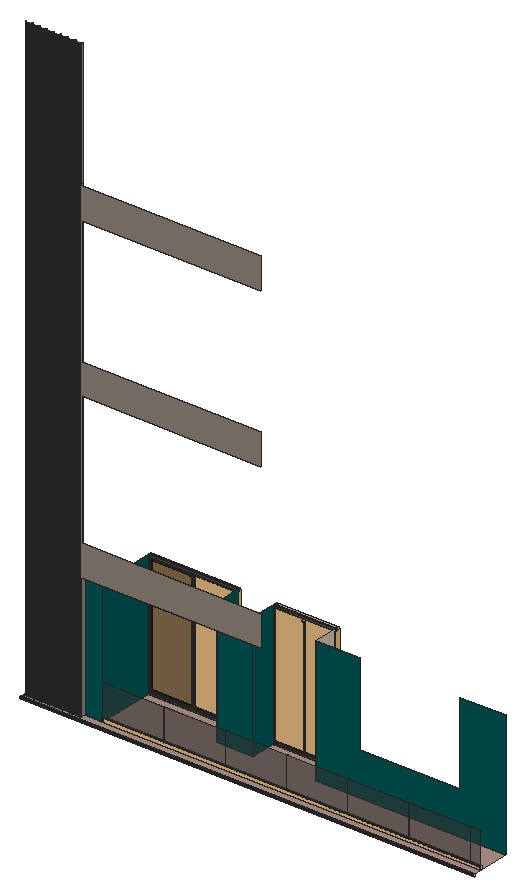
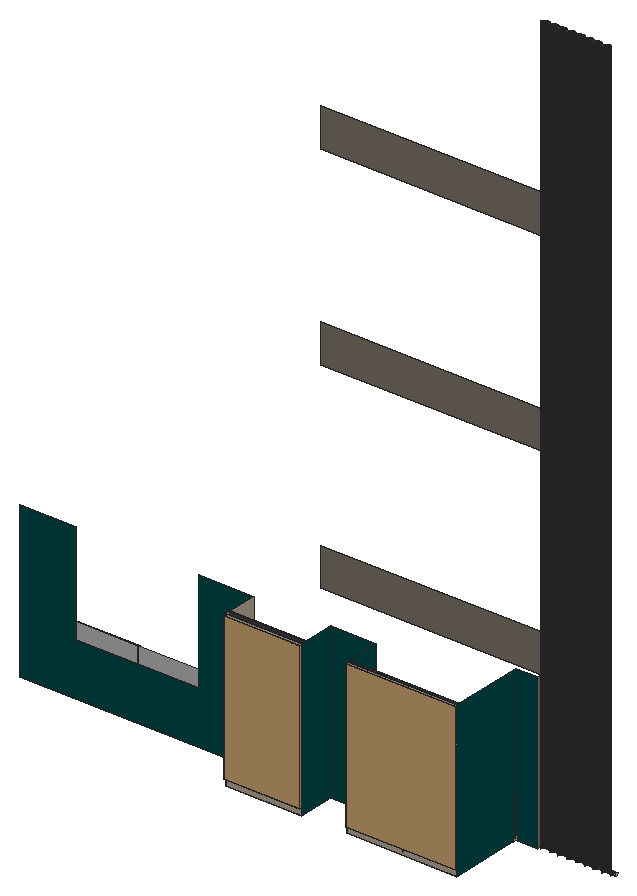
# SketchUp Ruby script. Lengths in inches.
U = 1.inch
M = Sketchup.active_model
def pt(a) = Geom::Point3d.new(a.map { |v| v * U })
def face(e, loops, mat)
  f = e.add_face(loops[0].map { |a| pt(a) })
  loops[1..].each { |l| e.add_face(l.map { |a| pt(a) }).erase! }
  f.material = f.back_material = mat if mat
  f
end
# faces: each face lists its corners as indices into pts; further lists are holes
def faces(e, pts, list, mat = nil) = list.each { |f| face(e, (f[0].is_a?(Array) ? f : [f]).map { |l| l.map { |i| pts[i] } }, mat) }
# xy, xz, yz: faces in a plane at the given z, y or x. An outline is a flat list of corners, or four numbers for a rectangle; further outlines are holes
def ring(l) = l.size == 4 ? [[l[0], l[1]], [l[2], l[1]], [l[2], l[3]], [l[0], l[3]]] : l.each_slice(2).to_a
def flat(e, list, mat, &to3) = list.each { |f| face(e, (f[0].is_a?(Array) ? f : [f]).map { |l| ring(l).map { |u, v| to3.(u, v) } }, mat) }
def xy(e, z, list, mat = nil) = flat(e, list, mat) { |x, y| [x, y, z] }
def xz(e, y, list, mat = nil) = flat(e, list, mat) { |x, z| [x, y, z] }
def yz(e, x, list, mat = nil) = flat(e, list, mat) { |y, z| [x, y, z] }
def lines(e, pts, list) = list.each { |a, b| e.add_line(pt(pts[a]), pt(pts[b])) }
# prism: a flat outline (further loops are holes) pulled along v
def prism(e, loops, v, mat = nil)
  f = face(e, loops, mat); d = Geom::Vector3d.new(v.map { |x| x * U })
  f.pushpull(f.normal.samedirection?(d) ? d.length : -d.length)
end
def box(e, o, s, mat = nil) = prism(e, [[o, [o[0] + s[0], o[1], o[2]], [o[0] + s[0], o[1] + s[1], o[2]], [o[0], o[1] + s[1], o[2]]]], [0, 0, s[2]], mat)
def at(x, y, z, deg = 0) = Geom::Transformation.translation(pt([x, y, z])) * Geom::Transformation.rotation(ORIGIN, Z_AXIS, deg.degrees)
def axes(o, x, y, z) = Geom::Transformation.new([*x, 0, *y, 0, *z, 0, *pt(o).to_a, 1])
def part(name) = M.definitions.add(name)
# library, detail: a bought-in or finely detailed component or shape, given as its bounding box
def library(name, o, s) = part(name).tap { |d| box(d.entities, o, s) }
def detail(e, o, s) = box(e.add_group.entities, o, s)
def put(e, d, t, mat = nil) = e.add_instance(d, t).tap { |i| i.material = mat if mat }
def group(e, t, mat = nil) = e.add_group.tap { |g| g.transformation = t; g.material = mat if mat }.entities
root = M.entities
M.materials.add("Brown Tiles 240cm").color = [174, 145, 135]
M.materials.add("Glass_Tinted_Gray").color = [0, 0, 0]
M.materials["Glass_Tinted_Gray"].alpha = 0.125
M.materials.add("Heather_Band").color = [142, 133, 122]
M.materials.add("Lily_Blonde").color = [209, 194, 173]
M.materials.add("[0135_DarkGray]").color = [81, 81, 81]
M.materials.add("[Color H08]").color = [0, 84, 84]
M.materials.add("[Mirror 02]").color = [229, 229, 229]
M.materials.add("[Terrazzo Light Blue]").color = [196, 214, 227]
M.materials.add("[Translucent_Glass_Blue]").color = [63, 63, 63]
M.materials["[Translucent_Glass_Blue]"].alpha = 0.35
M.materials.add("metal railing").color = [165, 165, 165]
M.materials.add("plastic2").color = [86, 86, 86]
c1 = library("Window curtains",[0,0,0],[14.46,147.43,135.83])
c2 = part("PENTEK_RP Fineline 50S_Sliding_DoorCase_E1")
box(c2.entities,[0,0,0],[1.51,3.66,99.27],"[0135_DarkGray]")
c3 = part("PENTEK_RP Fineline 50S_SlidingDooe_Case_E2")
box(c3.entities,[0,0,0],[96.25,3.66,1.51],"[0135_DarkGray]")
c4 = part("pentek_RP Fineline 50S_SlidingDoor_Case")
put(c4.entities,c2,at(97.76,0,0))
put(c4.entities,c3,at(1.51,0,0))
put(c4.entities,c2,at(0,0,0))
put(c4.entities,c3,at(1.51,0,97.76))
c5 = part("PENTEK_RP Fineline 50S_SlidingDoor_GlazingBead_2")
box(c5.entities,[0,0,0],[0.56,0.59,94.39],"[0135_DarkGray]")
c6 = part("PENTEK_RP Fineline 50S_SlidingDoor_Glass")
box(c6.entities,[0,0,0],[46.58,0.16,94.39],"Glass_Tinted_Gray")
c7 = part("PENTEK_RP Fineline 50S_SlidingDoor_GlazingBead")
box(c7.entities,[0,0,0],[45.47,0.59,0.56],"[0135_DarkGray]")
c8 = part("PENTEK_RP Fineline 50S_SlidingDoor_Leaf_E1")
xy(c8.entities,0,[[0,0,0.93,1.97],[0.93,1.57,1.49,1.97]],"[0135_DarkGray]")
xy(c8.entities,96.25,[[0,0,0.93,0,0.93,1.57,1.49,1.57,1.49,1.97,0,1.97]],"[0135_DarkGray]")
xz(c8.entities,0,[[0,0,0.93,96.25]],"[0135_DarkGray]")
xz(c8.entities,1.57,[[0.93,0,1.49,95.32],[0.93,95.32,1.49,96.25]],"[0135_DarkGray]")
xz(c8.entities,1.97,[[0,0,1.49,96.25]],"[0135_DarkGray]")
yz(c8.entities,0,[[0,0,1.97,96.25]],"[0135_DarkGray]")
yz(c8.entities,0.93,[[0,0,1.57,0.93],[0,0.93,1.57,95.32],[0,95.32,1.57,96.25]],"[0135_DarkGray]")
yz(c8.entities,1.49,[[1.57,0,1.97,95.32],[1.57,95.32,1.97,96.25]],"[0135_DarkGray]")
c9 = part("PENTEK_RP Fineline 50S_SlidingDoor_Leaf_E2")
xy(c9.entities,0,[[0,0,0,1.57,0.56,1.57,0.56,1.97,46.02,1.97,46.02,1.57,46.58,1.57,46.58,0]],"[0135_DarkGray]")
xy(c9.entities,0.93,[[0,0,46.58,1.57]],"[0135_DarkGray]")
xy(c9.entities,1.49,[[0.56,1.57,46.02,1.97]],"[0135_DarkGray]")
xz(c9.entities,0,[[0,0,46.58,0.93]],"[0135_DarkGray]")
xz(c9.entities,1.57,[[0,0,0.56,0.93],[46.02,0,46.58,0.93],[0.56,0.93,46.02,1.49]],"[0135_DarkGray]")
xz(c9.entities,1.97,[[0.56,0,46.02,1.49]],"[0135_DarkGray]")
yz(c9.entities,0,[[0,0,1.57,0.93]],"[0135_DarkGray]")
yz(c9.entities,0.56,[[1.57,0,1.97,0.93],[1.57,0.93,1.97,1.49]],"[0135_DarkGray]")
yz(c9.entities,46.02,[[1.57,0,1.97,0.93],[1.57,0.93,1.97,1.49]],"[0135_DarkGray]")
yz(c9.entities,46.58,[[0,0,1.57,0.93]],"[0135_DarkGray]")
c10 = part("PENTEK_RP Fineline S_SlidingDoor_Leaf1")
put(c10.entities,c5,at(0.93,0,0.93))
put(c10.entities,c5,at(46.96,0,0.93))
put(c10.entities,c6,at(1.49,1.42,0.93))
put(c10.entities,c7,at(1.49,0,0.93))
put(c10.entities,c6,at(1.49,0.59,0.93),"[Terrazzo Light Blue]")
put(c10.entities,c8,at(0,0,0))
put(c10.entities,c8,axes([48.44,0,0],[-1,0,0],[0,1,0],[0,0,1]))
put(c10.entities,c9,axes([0.93,0,96.25],[1,0,0],[0,1,0],[0,0,-1]))
put(c10.entities,c9,at(0.93,0,0))
put(c10.entities,c7,at(1.49,0,94.77))
c11 = part("PENTEK_RP Fineline 50S_SlidingDoor_Leaf2")
put(c11.entities,c6,at(1.49,1.42,0.93))
put(c11.entities,c7,at(1.49,0,94.77))
put(c11.entities,c5,at(46.96,0,0.93))
put(c11.entities,c6,at(1.49,0.59,0.93),"[Mirror 02]")
put(c11.entities,c5,at(0.93,0,0.93))
put(c11.entities,c8,at(0,0,0))
put(c11.entities,c8,axes([48.44,0,0],[-1,0,0],[0,1,0],[0,0,1]))
put(c11.entities,c7,at(1.49,0,0.93))
put(c11.entities,c9,axes([0.93,0,96.25],[1,0,0],[0,1,0],[0,0,-1]))
put(c11.entities,c9,at(0.93,0,0))
c12 = part("PENTEK - Slimmest Steel Sliding Door / Window\#1")
put(c12.entities,c4,at(0,-1.88,-0.09))
put(c12.entities,c10,at(1.51,-2.27,1.42))
put(c12.entities,c11,at(49.32,-0.3,1.42))
c13 = library("Railing",[0,0,0],[72,2.52,4.03])
c14 = part("railing plastic")
box(c14.entities,[0,0.75,0],[72,0.26,0.68],"plastic2")
box(c14.entities,[0,0,0],[72,0.26,0.68],"plastic2")
c15 = part("Glass Railing pro")
put(c15.entities,c13,axes([0,0,0],[6.18776,0,0],[0,1,0],[0,0,1]))
put(c15.entities,c14,axes([0,0.75,3.47],[6.18776,0,0],[0,1,0],[0,0,1]))
c16 = part("sheet glass")
box(c16.entities,[0,0,0],[39.37,0.39,39.37],"[Translucent_Glass_Blue]")
c17 = part("glass stretch")
box(c17.entities,[0,0,0],[39.37,0.39,43.31],"[Translucent_Glass_Blue]")
c18 = part("glass frame")
put(c18.entities,c16,axes([0,0,0],[1.8288,0,0],[0,1.016,0],[0,0,1]))
put(c18.entities,c17,axes([433.2,0,0],[0.3129,0,0],[0,1.016,0],[0,0,0.90909]))
put(c18.entities,c16,axes([72.2,0,0],[1.8288,0,0],[0,1.016,0],[0,0,1]))
put(c18.entities,c16,axes([144.4,0,0],[1.8288,0,0],[0,1.016,0],[0,0,1]))
put(c18.entities,c16,axes([216.6,0,0],[1.8288,0,0],[0,1.016,0],[0,0,1]))
put(c18.entities,c16,axes([288.8,0,0],[1.8288,0,0],[0,1.016,0],[0,0,1]))
put(c18.entities,c16,axes([361,0,0],[1.8288,0,0],[0,1.016,0],[0,0,1]))
c19 = part("Glass Railing +")
put(c19.entities,c15,at(0,0,0),"metal railing")
put(c19.entities,c18,at(0,1.0625,1.53),"metal railing")
c20 = part("My+Glass_Railing")
put(c20.entities,c19,at(-0.29,0,0))
c21 = part("Group\#18")
put(c21.entities,c1,axes([0,8.14,5.43],[0,-0.42,0],[1.40442,0,0],[0,0,0.9702]))
put(c21.entities,c12,axes([0,2.27,0.13],[2.0736,0,0],[0,1,0],[0,0,1.4]))
xy(root,219.25,[[0,1.33,534.76,1.33,534.76,46.67,311.15,46.67,311.15,80.33,237.9,80.33,237.9,45.95,195.07,45.95,195.07,80.33,89.34,80.33,89.34,9.49,68.4,9.49,68.4,4.77,0,4.77]],"Brown Tiles 240cm")
xy(root,219.25,[[0,4.77,67.06,4.77,67.06,8.08,66.92,7.74,66.75,7.42,66.5625,7.11,66.35,6.82,66.11,6.54,65.85,6.29,65.57,6.06,65.27,5.85,64.96,5.66,64.63,5.51,64.29,5.375,63.94,5.27,63.59,5.2,63.23,5.16,62.86,5.14,62.5,5.16,62.14,5.2,61.79,5.27,61.4375,5.375,61.1,5.51,60.77,5.66,60.46,5.85,60.16,6.06,59.88,6.29,59.62,6.54,59.38,6.82,59.17,7.11,58.98,7.42,58.8125,7.74,58.67,8.08,58.54,7.74,58.37,7.42,58.18,7.11,57.97,6.82,57.73,6.54,57.47,6.29,57.1875,6.06,56.89,5.85,56.58,5.66,56.25,5.51,55.91,5.375,55.5625,5.27,55.21,5.2,54.85,5.16,54.48,5.14,54.12,5.16,53.76,5.2,53.4,5.27,53.05,5.375,52.72,5.51,52.39,5.66,52.07,5.85,51.78,6.06,51.5,6.29,51.24,6.54,51,6.82,50.78,7.11,50.59,7.42,50.43,7.74,50.29,8.08,50.15,7.74,49.99,7.42,49.8,7.11,49.58,6.82,49.35,6.54,49.09,6.29,48.81,6.06,48.51,5.85,48.2,5.66,47.87,5.51,47.53,5.375,47.18,5.27,46.82,5.2,46.46,5.16,46.1,5.14,45.74,5.16,45.375,5.2,45.02,5.27,44.67,5.375,44.33,5.51,44.01,5.66,43.69,5.85,43.39,6.06,43.12,6.29,42.86,6.54,42.62,6.82,42.4,7.11,42.21,7.42,42.05,7.74,41.91,8.08,41.77,7.74,41.61,7.42,41.42,7.11,41.2,6.82,40.96,6.54,40.7,6.29,40.42,6.06,40.125,5.85,39.8125,5.66,39.49,5.51,39.15,5.375,38.8,5.27,38.44,5.2,38.08,5.16,37.72,5.14,37.36,5.16,37,5.2,36.64,5.27,36.29,5.375,35.95,5.51,35.625,5.66,35.3125,5.85,35.01,6.06,34.73,6.29,34.47,6.54,34.24,6.82,34.02,7.11,33.83,7.42,33.67,7.74,33.53,8.08,33.39,7.74,33.23,7.42,33.03,7.11,32.82,6.82,32.58,6.54,32.32,6.29,32.04,6.06,31.74,5.85,31.43,5.66,31.1,5.51,30.76,5.375,30.42,5.27,30.06,5.2,29.7,5.16,29.34,5.14,28.97,5.16,28.61,5.2,28.26,5.27,27.91,5.375,27.57,5.51,27.24,5.66,26.93,5.85,26.63,6.06,26.35,6.29,26.09,6.54,25.85,6.82,25.64,7.11,25.45,7.42,25.28,7.74,25.15,8.08,25.01,7.74,24.84,7.42,24.65,7.11,24.4375,6.82,24.2,6.54,23.94,6.29,23.66,6.06,23.36,5.85,23.05,5.66,22.72,5.51,22.38,5.375,22.03,5.27,21.68,5.2,21.32,5.16,20.95,5.14,20.59,5.16,20.23,5.2,19.875,5.27,19.53,5.375,19.1875,5.51,18.86,5.66,18.55,5.85,18.25,6.06,17.97,6.29,17.71,6.54,17.47,6.82,17.26,7.11,17.07,7.42,16.9,7.74,16.76,8.08,16.625,7.74,16.46,7.42,16.27,7.11,16.06,6.82,15.82,6.54,15.56,6.29,15.28,6.06,14.98,5.85,14.67,5.66,14.34,5.51,14,5.375,13.65,5.27,13.3,5.2,12.9375,5.16,12.57,5.14,12.21,5.16,11.85,5.2,11.49,5.27,11.14,5.375,10.81,5.51,10.48,5.66,10.16,5.85,9.87,6.06,9.59,6.29,9.33,6.54,9.09,6.82,8.875,7.11,8.68,7.42,8.52,7.74,8.38,8.08,8.24,7.74,8.08,7.42,7.89,7.11,7.67,6.82,7.4375,6.54,7.18,6.29,6.9,6.06,6.6,5.85,6.29,5.66,5.96,5.51,5.62,5.375,5.27,5.27,4.91,5.2,4.55,5.16,4.19,5.14,3.83,5.16,3.47,5.2,3.11,5.27,2.76,5.375,2.42,5.51,2.1,5.66,1.78,5.85,1.49,6.06,1.21,6.29,0.95,6.54,0.71,6.82,0.49,7.11,0.3,7.42,0.14,7.74,0,8.08]],"Heather_Band")
xz(root,1.33,[[0,216.59,534.76,219.25]])
xz(root,4.77,[[67.06,219.25,68.4,219.25,68.4,366.625,279.88,366.625,279.88,403.08,68.4,403.08,68.4,558.33,279.88,558.33,279.88,594.72,68.4,594.72,68.4,743.26,279.88,743.26,279.88,780.59,67.06,780.59]],"Heather_Band")
xz(root,9.49,[[68.4,219.25,89.34,366.625]],"[Color H08]")
xz(root,45.95,[[195.07,219.25,237.9,366.625]],"[Color H08]")
xz(root,46.67,[[311.15,219.25,534.76,219.25,534.76,366.625,481.45,366.625,481.45,270.02,363.26,270.02,363.26,366.625,311.15,366.625]],"[Color H08]")
xz(root,80.33,[[89.34,219.25,195.07,366.625],[237.9,219.25,311.15,366.625]],"Lily_Blonde")
yz(root,0,[[1.33,216.59,1.15,216.61,0.98,216.64,0.82,216.69,0.66,216.77,0.52,216.87,0.39,216.98,0.27,217.11,0.18,217.26,0.1,217.41,0.05,217.58,0.01,217.75,0,217.92,0.01,218.1,0.05,218.27,0.1,218.43,0.18,218.59,0.27,218.73,0.39,218.86,0.52,218.98,0.66,219.07,0.82,219.15,0.98,219.2,1.15,219.24,1.33,219.25]])
yz(root,67.06,[[4.77,219.25,8.08,780.59]],"Heather_Band")
yz(root,68.4,[[4.77,219.25,9.49,366.625]],"Heather_Band")
yz(root,89.34,[[9.49,219.25,80.33,366.625]],"[Color H08]")
yz(root,195.07,[[45.95,219.25,80.33,366.625]],"[Color H08]")
yz(root,237.9,[[45.95,219.25,80.33,366.625]],"[Color H08]")
yz(root,311.15,[[46.67,219.25,80.33,366.625]],"Lily_Blonde")
yz(root,534.76,[[1.33,216.59,1.33,219.25,1.15,219.24,0.98,219.2,0.82,219.15,0.66,219.07,0.52,218.98,0.39,218.86,0.27,218.73,0.18,218.59,0.1,218.43,0.05,218.27,0.01,218.1,0,217.92,0.01,217.75,0.05,217.58,0.1,217.41,0.18,217.26,0.27,217.11,0.39,216.98,0.52,216.87,0.66,216.77,0.82,216.69,0.98,216.64,1.15,216.61]])
p = [[534.76,0.98,216.64],[534.76,0.82,216.69],[0,0.82,216.69],[0,0.98,216.64],[534.76,1.15,216.61],[0,1.15,216.61],
  [534.76,1.33,216.59],[0,1.33,216.59],[534.76,0.66,216.77],[0,0.66,216.77],[534.76,0.52,216.87],[0,0.52,216.87],
  [534.76,0.39,216.98],[0,0.39,216.98],[534.76,0.27,217.11],[0,0.27,217.11],[534.76,0.18,217.26],[0,0.18,217.26],
  [534.76,0.1,217.41],[0,0.1,217.41],[534.76,0.05,217.58],[0,0.05,217.58],[534.76,0.01,217.75],[0,0.01,217.75],
  [534.76,0,217.92],[0,0,217.92],[534.76,0.01,218.1],[0,0.01,218.1],[534.76,0.05,218.27],[0,0.05,218.27],
  [534.76,0.1,218.43],[0,0.1,218.43],[534.76,0.18,218.59],[0,0.18,218.59],[534.76,0.27,218.73],[0,0.27,218.73],
  [534.76,0.39,218.86],[0,0.39,218.86],[534.76,0.52,218.98],[0,0.52,218.98],[534.76,0.66,219.07],[0,0.66,219.07],
  [534.76,0.82,219.15],[0,0.82,219.15],[534.76,0.98,219.2],[0,0.98,219.2],[534.76,1.15,219.24],[0,1.15,219.24],
  [534.76,1.33,219.25],[0,1.33,219.25],[4.19,5.14,929.63],[3.83,5.16,929.63],[3.83,5.16,219.25],[4.19,5.14,219.25],
  [4.55,5.16,929.63],[4.55,5.16,219.25],[12.57,5.14,929.63],[12.21,5.16,929.63],[12.21,5.16,219.25],[12.57,5.14,219.25],
  [12.9375,5.16,929.63],[12.9375,5.16,219.25],[20.95,5.14,929.63],[20.59,5.16,929.63],[20.59,5.16,219.25],[20.95,5.14,219.25],
  [21.32,5.16,929.63],[21.32,5.16,219.25],[29.34,5.14,929.63],[28.97,5.16,929.63],[28.97,5.16,219.25],[29.34,5.14,219.25],
  [29.7,5.16,929.63],[29.7,5.16,219.25],[37.72,5.14,929.63],[37.36,5.16,929.63],[37.36,5.16,219.25],[37.72,5.14,219.25],
  [38.08,5.16,929.63],[38.08,5.16,219.25],[46.1,5.14,929.63],[45.74,5.16,929.63],[45.74,5.16,219.25],[46.1,5.14,219.25],
  [46.46,5.16,929.63],[46.46,5.16,219.25],[54.48,5.14,929.63],[54.12,5.16,929.63],[54.12,5.16,219.25],[54.48,5.14,219.25],
  [54.85,5.16,929.63],[54.85,5.16,219.25],[62.86,5.14,929.63],[62.5,5.16,929.63],[62.5,5.16,219.25],[62.86,5.14,219.25],
  [63.23,5.16,929.63],[63.23,5.16,219.25],[3.47,5.2,929.63],[3.11,5.27,929.63],[3.11,5.27,219.25],[3.47,5.2,219.25],
  [4.91,5.2,929.63],[4.91,5.2,219.25],[5.27,5.27,929.63],[5.27,5.27,219.25],[11.85,5.2,929.63],[11.49,5.27,929.63],
  [11.49,5.27,219.25],[11.85,5.2,219.25],[13.3,5.2,929.63],[13.3,5.2,219.25],[13.65,5.27,929.63],[13.65,5.27,219.25],
  [20.23,5.2,929.63],[19.875,5.27,929.63],[19.875,5.27,219.25],[20.23,5.2,219.25],[21.68,5.2,929.63],[21.68,5.2,219.25],
  [22.03,5.27,929.63],[22.03,5.27,219.25],[28.61,5.2,929.63],[28.26,5.27,929.63],[28.26,5.27,219.25],[28.61,5.2,219.25],
  [30.06,5.2,929.63],[30.06,5.2,219.25],[30.42,5.27,929.63],[30.42,5.27,219.25],[37,5.2,929.63],[36.64,5.27,929.63],
  [36.64,5.27,219.25],[37,5.2,219.25],[38.44,5.2,929.63],[38.44,5.2,219.25],[38.8,5.27,929.63],[38.8,5.27,219.25],
  [45.375,5.2,929.63],[45.02,5.27,929.63],[45.02,5.27,219.25],[45.375,5.2,219.25],[46.82,5.2,929.63],[46.82,5.2,219.25],
  [47.18,5.27,929.63],[47.18,5.27,219.25],[53.76,5.2,929.63],[53.4,5.27,929.63],[53.4,5.27,219.25],[53.76,5.2,219.25],
  [55.21,5.2,929.63],[55.21,5.2,219.25],[55.5625,5.27,929.63],[55.5625,5.27,219.25],[62.14,5.2,929.63],[61.79,5.27,929.63],
  [61.79,5.27,219.25],[62.14,5.2,219.25],[63.59,5.2,929.63],[63.59,5.2,219.25],[63.94,5.27,929.63],[63.94,5.27,219.25],
  [2.76,5.375,929.63],[2.76,5.375,219.25],[5.62,5.375,929.63],[5.62,5.375,219.25],[11.14,5.375,929.63],[11.14,5.375,219.25],
  [14,5.375,929.63],[14,5.375,219.25],[19.53,5.375,929.63],[19.53,5.375,219.25],[22.38,5.375,929.63],[22.38,5.375,219.25],
  [27.91,5.375,929.63],[27.91,5.375,219.25],[30.76,5.375,929.63],[30.76,5.375,219.25],[36.29,5.375,929.63],[36.29,5.375,219.25],
  [39.15,5.375,929.63],[39.15,5.375,219.25],[44.67,5.375,929.63],[44.67,5.375,219.25],[47.53,5.375,929.63],[47.53,5.375,219.25],
  [53.05,5.375,929.63],[53.05,5.375,219.25],[55.91,5.375,929.63],[55.91,5.375,219.25],[61.4375,5.375,929.63],[61.4375,5.375,219.25],
  [64.29,5.375,929.63],[64.29,5.375,219.25],[2.42,5.51,929.63],[2.42,5.51,219.25],[5.96,5.51,929.63],[5.96,5.51,219.25],
  [10.81,5.51,929.63],[10.81,5.51,219.25],[14.34,5.51,929.63],[14.34,5.51,219.25],[19.1875,5.51,929.63],[19.1875,5.51,219.25],
  [22.72,5.51,929.63],[22.72,5.51,219.25],[27.57,5.51,929.63],[27.57,5.51,219.25],[31.1,5.51,929.63],[31.1,5.51,219.25],
  [35.95,5.51,929.63],[35.95,5.51,219.25],[39.49,5.51,929.63],[39.49,5.51,219.25],[44.33,5.51,929.63],[44.33,5.51,219.25],
  [47.87,5.51,929.63],[47.87,5.51,219.25],[52.72,5.51,929.63],[52.72,5.51,219.25],[56.25,5.51,929.63],[56.25,5.51,219.25],
  [61.1,5.51,929.63],[61.1,5.51,219.25],[64.63,5.51,929.63],[64.63,5.51,219.25],[2.1,5.66,929.63],[2.1,5.66,219.25],
  [6.29,5.66,929.63],[6.29,5.66,219.25],[10.48,5.66,929.63],[10.48,5.66,219.25],[14.67,5.66,929.63],[14.67,5.66,219.25],
  [18.86,5.66,929.63],[18.86,5.66,219.25],[23.05,5.66,929.63],[23.05,5.66,219.25],[27.24,5.66,929.63],[27.24,5.66,219.25],
  [31.43,5.66,929.63],[31.43,5.66,219.25],[35.625,5.66,929.63],[35.625,5.66,219.25],[39.8125,5.66,929.63],[39.8125,5.66,219.25],
  [44.01,5.66,929.63],[44.01,5.66,219.25],[48.2,5.66,929.63],[48.2,5.66,219.25],[52.39,5.66,929.63],[52.39,5.66,219.25],
  [56.58,5.66,929.63],[56.58,5.66,219.25],[60.77,5.66,929.63],[60.77,5.66,219.25],[64.96,5.66,929.63],[64.96,5.66,219.25],
  [1.78,5.85,929.63],[1.78,5.85,219.25],[6.6,5.85,929.63],[6.6,5.85,219.25],[10.16,5.85,929.63],[10.16,5.85,219.25],
  [14.98,5.85,929.63],[14.98,5.85,219.25],[18.55,5.85,929.63],[18.55,5.85,219.25],[23.36,5.85,929.63],[23.36,5.85,219.25],
  [26.93,5.85,929.63],[26.93,5.85,219.25],[31.74,5.85,929.63],[31.74,5.85,219.25],[35.3125,5.85,929.63],[35.3125,5.85,219.25],
  [40.125,5.85,929.63],[40.125,5.85,219.25],[43.69,5.85,929.63],[43.69,5.85,219.25],[48.51,5.85,929.63],[48.51,5.85,219.25],
  [52.07,5.85,929.63],[52.07,5.85,219.25],[56.89,5.85,929.63],[56.89,5.85,219.25],[60.46,5.85,929.63],[60.46,5.85,219.25],
  [65.27,5.85,929.63],[65.27,5.85,219.25],[1.49,6.06,929.63],[1.49,6.06,219.25],[6.9,6.06,929.63],[6.9,6.06,219.25],
  [9.87,6.06,929.63],[9.87,6.06,219.25],[15.28,6.06,929.63],[15.28,6.06,219.25],[18.25,6.06,929.63],[18.25,6.06,219.25],
  [23.66,6.06,929.63],[23.66,6.06,219.25],[26.63,6.06,929.63],[26.63,6.06,219.25],[32.04,6.06,929.63],[32.04,6.06,219.25],
  [35.01,6.06,929.63],[35.01,6.06,219.25],[40.42,6.06,929.63],[40.42,6.06,219.25],[43.39,6.06,929.63],[43.39,6.06,219.25],
  [48.81,6.06,929.63],[48.81,6.06,219.25],[51.78,6.06,929.63],[51.78,6.06,219.25],[57.1875,6.06,929.63],[57.1875,6.06,219.25],
  [60.16,6.06,929.63],[60.16,6.06,219.25],[65.57,6.06,929.63],[65.57,6.06,219.25],[1.21,6.29,929.63],[1.21,6.29,219.25],
  [7.18,6.29,929.63],[7.18,6.29,219.25],[9.59,6.29,929.63],[9.59,6.29,219.25],[15.56,6.29,929.63],[15.56,6.29,219.25],
  [17.97,6.29,929.63],[17.97,6.29,219.25],[23.94,6.29,929.63],[23.94,6.29,219.25],[26.35,6.29,929.63],[26.35,6.29,219.25],
  [32.32,6.29,929.63],[32.32,6.29,219.25],[34.73,6.29,929.63],[34.73,6.29,219.25],[40.7,6.29,929.63],[40.7,6.29,219.25],
  [43.12,6.29,929.63],[43.12,6.29,219.25],[49.09,6.29,929.63],[49.09,6.29,219.25],[51.5,6.29,929.63],[51.5,6.29,219.25],
  [57.47,6.29,929.63],[57.47,6.29,219.25],[59.88,6.29,929.63],[59.88,6.29,219.25],[65.85,6.29,929.63],[65.85,6.29,219.25],
  [0.95,6.54,929.63],[0.95,6.54,219.25],[7.4375,6.54,929.63],[7.4375,6.54,219.25],[9.33,6.54,929.63],[9.33,6.54,219.25],
  [15.82,6.54,929.63],[15.82,6.54,219.25],[17.71,6.54,929.63],[17.71,6.54,219.25],[24.2,6.54,929.63],[24.2,6.54,219.25],
  [26.09,6.54,929.63],[26.09,6.54,219.25],[32.58,6.54,929.63],[32.58,6.54,219.25],[34.47,6.54,929.63],[34.47,6.54,219.25],
  [40.96,6.54,929.63],[40.96,6.54,219.25],[42.86,6.54,929.63],[42.86,6.54,219.25],[49.35,6.54,929.63],[49.35,6.54,219.25],
  [51.24,6.54,929.63],[51.24,6.54,219.25],[57.73,6.54,929.63],[57.73,6.54,219.25],[59.62,6.54,929.63],[59.62,6.54,219.25],
  [66.11,6.54,929.63],[66.11,6.54,219.25],[0.71,6.82,929.63],[0.71,6.82,219.25],[7.67,6.82,929.63],[7.67,6.82,219.25],
  [9.09,6.82,929.63],[9.09,6.82,219.25],[16.06,6.82,929.63],[16.06,6.82,219.25],[17.47,6.82,929.63],[17.47,6.82,219.25],
  [24.4375,6.82,929.63],[24.4375,6.82,219.25],[25.85,6.82,929.63],[25.85,6.82,219.25],[32.82,6.82,929.63],[32.82,6.82,219.25],
  [34.24,6.82,929.63],[34.24,6.82,219.25],[41.2,6.82,929.63],[41.2,6.82,219.25],[42.62,6.82,929.63],[42.62,6.82,219.25],
  [49.39,6.59,929.63],[49.58,6.82,219.25],[49.58,6.82,929.63],[51,6.82,929.63],[51,6.82,219.25],[57.97,6.82,929.63],
  [57.97,6.82,219.25],[59.38,6.82,929.63],[59.38,6.82,219.25],[66.35,6.82,929.63],[66.35,6.82,219.25],[0.49,7.11,929.63],
  [0.49,7.11,219.25],[7.89,7.11,929.63],[7.89,7.11,219.25],[8.875,7.11,929.63],[8.875,7.11,219.25],[16.27,7.11,929.63],
  [16.27,7.11,219.25],[17.26,7.11,929.63],[17.26,7.11,219.25],[24.65,7.11,929.63],[24.65,7.11,219.25],[25.64,7.11,929.63],
  [25.64,7.11,219.25],[33.03,7.11,929.63],[33.03,7.11,219.25],[34.02,7.11,929.63],[34.02,7.11,219.25],[41.42,7.11,929.63],
  [41.42,7.11,219.25],[42.4,7.11,929.63],[42.4,7.11,219.25],[49.8,7.11,929.63],[49.8,7.11,219.25],[50.78,7.11,929.63],
  [50.78,7.11,219.25],[58.18,7.11,929.63],[58.18,7.11,219.25],[59.17,7.11,929.63],[59.17,7.11,219.25],[66.5625,7.11,929.63],
  [66.5625,7.11,219.25],[0.3,7.42,929.63],[0.3,7.42,219.25],[8.08,7.42,929.63],[8.08,7.42,219.25],[8.68,7.42,929.63],
  [8.68,7.42,219.25],[16.46,7.42,929.63],[16.46,7.42,219.25],[17.07,7.42,929.63],[17.07,7.42,219.25],[24.84,7.42,929.63],
  [24.84,7.42,219.25],[25.45,7.42,929.63],[25.45,7.42,219.25],[33.23,7.42,929.63],[33.23,7.42,219.25],[33.83,7.42,929.63],
  [33.83,7.42,219.25],[41.61,7.42,929.63],[41.61,7.42,219.25],[42.21,7.42,929.63],[42.21,7.42,219.25],[49.99,7.42,929.63],
  [49.99,7.42,219.25],[50.59,7.42,929.63],[50.59,7.42,219.25],[58.37,7.42,929.63],[58.37,7.42,219.25],[58.98,7.42,929.63],
  [58.98,7.42,219.25],[66.75,7.42,929.63],[66.75,7.42,219.25],[0.14,7.74,929.63],[0.14,7.74,219.25],[8.24,7.74,929.63],
  [8.24,7.74,219.25],[8.52,7.74,929.63],[8.52,7.74,219.25],[16.625,7.74,929.63],[16.625,7.74,219.25],[16.9,7.74,929.63],
  [16.9,7.74,219.25],[25.01,7.74,929.63],[25.01,7.74,219.25],[25.28,7.74,929.63],[25.28,7.74,219.25],[33.39,7.74,929.63],
  [33.39,7.74,219.25],[33.67,7.74,929.63],[33.67,7.74,219.25],[41.77,7.74,929.63],[41.77,7.74,219.25],[42.05,7.74,929.63],
  [42.05,7.74,219.25],[50.15,7.74,929.63],[50.15,7.74,219.25],[50.43,7.74,929.63],[50.43,7.74,219.25],[58.54,7.74,929.63],
  [58.54,7.74,219.25],[58.8125,7.74,929.63],[58.8125,7.74,219.25],[66.92,7.74,929.63],[66.92,7.74,219.25],[0,8.08,929.63],
  [0,8.08,926.45],[0,8.08,219.25],[8.38,8.08,929.63],[8.38,8.08,219.25],[8.38,8.08,926.45],[16.76,8.08,929.63],
  [16.76,8.08,219.25],[16.76,8.08,926.45],[25.15,8.08,929.63],[25.15,8.08,219.25],[25.15,8.08,926.45],[33.53,8.08,929.63],
  [33.53,8.08,219.25],[33.53,8.08,926.45],[41.91,8.08,929.63],[41.91,8.08,219.25],[41.91,8.08,926.45],[50.29,8.08,929.63],
  [50.29,8.08,219.25],[50.29,8.08,926.45],[58.67,8.08,929.63],[58.67,8.08,219.25],[58.67,8.08,926.45],[67.06,8.08,929.63],
  [67.06,8.08,219.25],[67.06,8.08,780.59],[67.06,8.08,926.45]]
faces(root,p,[[0,1,2,3],[4,0,3,5],[6,4,5,7],[1,8,9,2],[8,10,11,9],[10,12,13,11],[12,14,15,13],[14,16,17,15],
  [16,18,19,17],[18,20,21,19],[20,22,23,21],[22,24,25,23],[24,26,27,25],[26,28,29,27],[28,30,31,29],[30,32,33,31],
  [32,34,35,33],[34,36,37,35],[36,38,39,37],[38,40,41,39],[40,42,43,41],[42,44,45,43],[44,46,47,45],[46,48,49,47]],"[Color H08]")
faces(root,p,[[50,51,52,53],[54,50,53,55],[56,57,58,59],[60,56,59,61],[62,63,64,65],[66,62,65,67],[68,69,70,71],[72,68,71,73],
  [74,75,76,77],[78,74,77,79],[80,81,82,83],[84,80,83,85],[86,87,88,89],[90,86,89,91],[92,93,94,95],[96,92,95,97],
  [98,99,100,101],[51,98,101,52],[102,54,55,103],[104,102,103,105],[106,107,108,109],[57,106,109,58],[110,60,61,111],[112,110,111,113],
  [114,115,116,117],[63,114,117,64],[118,66,67,119],[120,118,119,121],[122,123,124,125],[69,122,125,70],[126,72,73,127],[128,126,127,129],
  [130,131,132,133],[75,130,133,76],[134,78,79,135],[136,134,135,137],[138,139,140,141],[81,138,141,82],[142,84,85,143],[144,142,143,145],
  [146,147,148,149],[87,146,149,88],[150,90,91,151],[152,150,151,153],[154,155,156,157],[93,154,157,94],[158,96,97,159],[160,158,159,161],
  [99,162,163,100],[164,104,105,165],[107,166,167,108],[168,112,113,169],[115,170,171,116],[172,120,121,173],[123,174,175,124],[176,128,129,177],
  [131,178,179,132],[180,136,137,181],[139,182,183,140],[184,144,145,185],[147,186,187,148],[188,152,153,189],[155,190,191,156],[192,160,161,193],
  [162,194,195,163],[196,164,165,197],[166,198,199,167],[200,168,169,201],[170,202,203,171],[204,172,173,205],[174,206,207,175],[208,176,177,209],
  [178,210,211,179],[212,180,181,213],[182,214,215,183],[216,184,185,217],[186,218,219,187],[220,188,189,221],[190,222,223,191],[224,192,193,225],
  [194,226,227,195],[228,196,197,229],[198,230,231,199],[232,200,201,233],[202,234,235,203],[236,204,205,237],[206,238,239,207],[240,208,209,241],
  [210,242,243,211],[244,212,213,245],[214,246,247,215],[248,216,217,249],[218,250,251,219],[252,220,221,253],[222,254,255,223],[256,224,225,257],
  [226,258,259,227],[260,228,229,261],[230,262,263,231],[264,232,233,265],[234,266,267,235],[268,236,237,269],[238,270,271,239],[272,240,241,273],
  [242,274,275,243],[276,244,245,277],[246,278,279,247],[280,248,249,281],[250,282,283,251],[284,252,253,285],[254,286,287,255],[288,256,257,289],
  [258,290,291,259],[292,260,261,293],[262,294,295,263],[296,264,265,297],[266,298,299,267],[300,268,269,301],[270,302,303,271],[304,272,273,305],
  [274,306,307,275],[308,276,277,309],[278,310,311,279],[312,280,281,313],[282,314,315,283],[316,284,285,317],[286,318,319,287],[320,288,289,321],
  [290,322,323,291],[324,292,293,325],[294,326,327,295],[328,296,297,329],[298,330,331,299],[332,300,301,333],[302,334,335,303],[336,304,305,337],
  [306,338,339,307],[340,308,309,341],[310,342,343,311],[344,312,313,345],[314,346,347,315],[348,316,317,349],[318,350,351,319],[352,320,321,353],
  [322,354,355,323],[356,324,325,357],[326,358,359,327],[360,328,329,361],[330,362,363,331],[364,332,333,365],[334,366,367,335],[368,336,337,369],
  [338,370,371,339],[372,340,341,373],[342,374,375,343],[376,344,345,377],[346,378,379,347],[380,348,349,381],[350,382,383,351],[384,352,353,385],
  [354,386,387,355],[388,356,357,389],[358,390,391,359],[392,360,361,393],[362,394,395,363],[396,364,365,397],[366,398,399,367],[400,368,369,401],
  [370,402,403,371],[404,372,373,405],[374,406,407,375],[408,376,377,409,410],[378,411,412,379],[413,380,381,414],[382,415,416,383],[417,384,385,418],
  [386,419,420,387],[421,388,389,422],[390,423,424,391],[425,392,393,426],[394,427,428,395],[429,396,397,430],[398,431,432,399],[433,400,401,434],
  [402,435,436,403],[437,404,405,438],[406,439,440,407],[441,410,409,442],[411,443,444,412],[445,413,414,446],[415,447,448,416],[449,417,418,450],
  [419,451,452,420],[453,421,422,454],[423,455,456,424],[457,425,426,458],[427,459,460,428],[461,429,430,462],[431,463,464,432],[465,433,434,466],
  [435,467,468,436],[469,437,438,470],[439,471,472,440],[473,441,442,474],[443,475,476,444],[477,445,446,478],[447,479,480,448],[481,449,450,482],
  [451,483,484,452],[485,453,454,486],[455,487,488,456],[489,457,458,490],[459,491,492,460],[493,461,462,494],[463,495,496,464],[497,465,466,498],
  [467,499,500,468],[501,469,470,502],[471,503,504,472],[505,473,474,506],[475,507,508,476],[509,477,478,510],[479,511,512,480],[513,481,482,514],
  [483,515,516,517,484],[518,485,486,519,520],[487,518,520,519,488],[521,489,490,522,523],[491,521,523,522,492],[524,493,494,525,526],[495,524,526,525,496],[527,497,498,528,529],
  [499,527,529,528,500],[530,501,502,531,532],[503,530,532,531,504],[533,505,506,534,535],[507,533,535,534,508],[536,509,510,537,538],[511,536,538,537,512],[539,513,514,540,541,542]],"Heather_Band")
g1 = group(root,at(239.43,71.53,219.25))
put(g1,c1,axes([0,9.375,5.76],[0,-0.48393,0],[0.49686,0,0],[0,0,1.0288]))
put(g1,c12,axes([0,3.99,0.14],[0.73361,0,0],[0,0.38023,0],[0,0,1.48455]))
put(root,c20,at(89.53,9.49,219.25))
put(root,c21,axes([89.34,77.1875,219.25],[0.51267,0,0],[0,0.5,0],[0,0,1.0604]))
